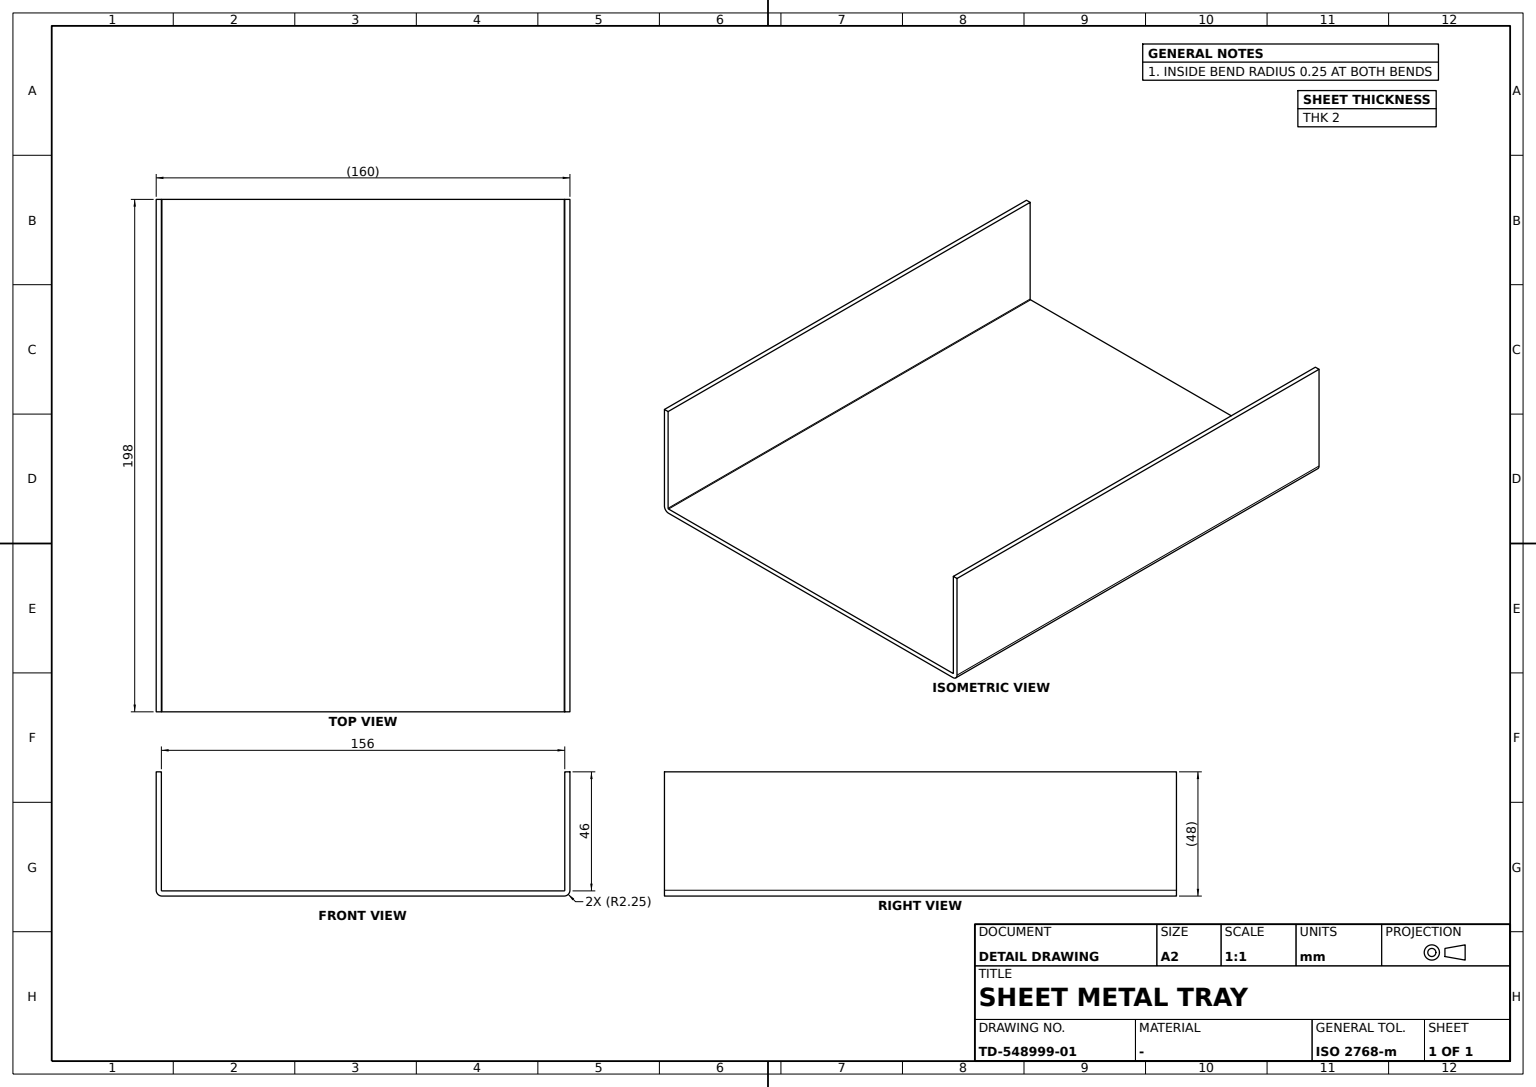
ISO-10303-21;
HEADER;
FILE_DESCRIPTION((''),'2;1');
FILE_NAME('','',(''),(''),'','','');
FILE_SCHEMA(('AUTOMOTIVE_DESIGN'));
ENDSEC;
DATA;
#1=APPLICATION_CONTEXT('');
#2=PRODUCT_CONTEXT('',#1,'mechanical');
#3=PRODUCT('','','',(#2));
#4=PRODUCT_DEFINITION_FORMATION('','',#3);
#5=PRODUCT_DEFINITION_CONTEXT('',#1,'design');
#6=PRODUCT_DEFINITION('','',#4,#5);
#7=PRODUCT_DEFINITION_SHAPE('','',#6);
#8=(LENGTH_UNIT()NAMED_UNIT(*)SI_UNIT(.MILLI.,.METRE.));
#9=(NAMED_UNIT(*)PLANE_ANGLE_UNIT()SI_UNIT($,.RADIAN.));
#10=(NAMED_UNIT(*)SI_UNIT($,.STERADIAN.)SOLID_ANGLE_UNIT());
#11=UNCERTAINTY_MEASURE_WITH_UNIT(LENGTH_MEASURE(1.E-05),#8,'distance_accuracy_value','');
#12=(GEOMETRIC_REPRESENTATION_CONTEXT(3)GLOBAL_UNCERTAINTY_ASSIGNED_CONTEXT((#11))GLOBAL_UNIT_ASSIGNED_CONTEXT((#8,#9,#10))REPRESENTATION_CONTEXT('',''));
#13=CARTESIAN_POINT('',(-77.75,-99.,0.));
#14=VERTEX_POINT('',#13);
#15=CARTESIAN_POINT('',(-80.,-99.,2.25));
#16=VERTEX_POINT('',#15);
#17=CARTESIAN_POINT('',(-77.75,-99.,2.25));
#18=DIRECTION('',(0.,1.,0.));
#19=DIRECTION('',(0.,0.,-1.));
#20=AXIS2_PLACEMENT_3D('',#17,#18,#19);
#21=CIRCLE('',#20,2.25);
#22=EDGE_CURVE('',#14,#16,#21,.T.);
#23=ORIENTED_EDGE('',*,*,#22,.F.);
#24=CARTESIAN_POINT('',(-77.75,-99.,2.));
#25=VERTEX_POINT('',#24);
#26=CARTESIAN_POINT('',(-77.75,-99.,1.));
#27=DIRECTION('',(0.,0.,1.));
#28=VECTOR('',#27,1000.);
#29=LINE('',#26,#28);
#30=EDGE_CURVE('',#14,#25,#29,.T.);
#31=ORIENTED_EDGE('',*,*,#30,.T.);
#32=CARTESIAN_POINT('',(-78.,-99.,2.25));
#33=VERTEX_POINT('',#32);
#34=CIRCLE('',#20,0.25);
#35=EDGE_CURVE('',#25,#33,#34,.T.);
#36=ORIENTED_EDGE('',*,*,#35,.T.);
#37=CARTESIAN_POINT('',(-79.,-99.,2.25));
#38=DIRECTION('',(1.,0.,0.));
#39=VECTOR('',#38,1000.);
#40=LINE('',#37,#39);
#41=EDGE_CURVE('',#16,#33,#40,.T.);
#42=ORIENTED_EDGE('',*,*,#41,.F.);
#43=EDGE_LOOP('',(#23,#31,#36,#42));
#44=FACE_OUTER_BOUND('',#43,.T.);
#45=CARTESIAN_POINT('',(-77.797124,-99.,2.));
#46=CARTESIAN_POINT('',(-78.174115,-99.,0.));
#47=CARTESIAN_POINT('',(-77.84425,-99.,2.011098));
#48=CARTESIAN_POINT('',(-78.59825,-99.,0.099885));
#49=CARTESIAN_POINT('',(-77.887876,-99.,2.03333));
#50=CARTESIAN_POINT('',(-78.990881,-99.,0.299966));
#51=CARTESIAN_POINT('',(-77.949009,-99.,2.085996));
#52=CARTESIAN_POINT('',(-79.541079,-99.,0.773968));
#53=CARTESIAN_POINT('',(-77.985194,-99.,2.156785));
#54=CARTESIAN_POINT('',(-79.866749,-99.,1.411067));
#55=CARTESIAN_POINT('',(-77.995066,-99.,2.187168));
#56=CARTESIAN_POINT('',(-79.955592,-99.,1.684512));
#57=CARTESIAN_POINT('',(-78.,-99.,2.218584));
#58=CARTESIAN_POINT('',(-80.,-99.,1.967257));
#59=B_SPLINE_SURFACE_WITH_KNOTS('',5,1,((#24,#13),(#45,#46),(#47,#48),(#49,#50),(#51,#52),(#53,#54),(#55,#56),(#57,#58),(#32,#15)),.UNSPECIFIED.,.F.,.F.,.F.,(6,3,6),(2,2),(0.,2.120575041,3.534291735),(-2.,0.),.UNSPECIFIED.);
#60=ADVANCED_FACE('',(#44),#59,.T.);
#61=CARTESIAN_POINT('',(80.,99.,2.25));
#62=VERTEX_POINT('',#61);
#63=CARTESIAN_POINT('',(78.,99.,2.25));
#64=VERTEX_POINT('',#63);
#65=CARTESIAN_POINT('',(79.,99.,2.25));
#66=DIRECTION('',(-1.,0.,0.));
#67=VECTOR('',#66,1000.);
#68=LINE('',#65,#67);
#69=EDGE_CURVE('',#62,#64,#68,.T.);
#70=ORIENTED_EDGE('',*,*,#69,.T.);
#71=CARTESIAN_POINT('',(78.,99.,48.));
#72=VERTEX_POINT('',#71);
#73=CARTESIAN_POINT('',(78.,99.,25.125));
#74=LINE('',#73,#28);
#75=EDGE_CURVE('',#64,#72,#74,.T.);
#76=ORIENTED_EDGE('',*,*,#75,.T.);
#77=CARTESIAN_POINT('',(80.,99.,48.));
#78=VERTEX_POINT('',#77);
#79=CARTESIAN_POINT('',(79.,99.,48.));
#80=LINE('',#79,#67);
#81=EDGE_CURVE('',#78,#72,#80,.T.);
#82=ORIENTED_EDGE('',*,*,#81,.F.);
#83=CARTESIAN_POINT('',(80.,99.,25.125));
#84=LINE('',#83,#28);
#85=EDGE_CURVE('',#62,#78,#84,.T.);
#86=ORIENTED_EDGE('',*,*,#85,.F.);
#87=EDGE_LOOP('',(#70,#76,#82,#86));
#88=FACE_OUTER_BOUND('',#87,.T.);
#89=CARTESIAN_POINT('',(78.,99.,2.));
#90=AXIS2_PLACEMENT_3D('',#89,#18,#27);
#91=PLANE('',#90);
#92=ADVANCED_FACE('',(#88),#91,.T.);
#93=CARTESIAN_POINT('',(-78.,99.,2.25));
#94=VERTEX_POINT('',#93);
#95=CARTESIAN_POINT('',(-78.,0.,2.25));
#96=DIRECTION('',(0.,-1.,0.));
#97=VECTOR('',#96,1000.);
#98=LINE('',#95,#97);
#99=EDGE_CURVE('',#94,#33,#98,.T.);
#100=ORIENTED_EDGE('',*,*,#99,.T.);
#101=ORIENTED_EDGE('',*,*,#35,.F.);
#102=CARTESIAN_POINT('',(-77.75,99.,2.));
#103=VERTEX_POINT('',#102);
#104=CARTESIAN_POINT('',(-77.75,0.,2.));
#105=VECTOR('',#18,1000.);
#106=LINE('',#104,#105);
#107=EDGE_CURVE('',#25,#103,#106,.T.);
#108=ORIENTED_EDGE('',*,*,#107,.T.);
#109=CARTESIAN_POINT('',(-77.75,99.,2.25));
#110=AXIS2_PLACEMENT_3D('',#109,#96,#19);
#111=CIRCLE('',#110,0.25);
#112=EDGE_CURVE('',#94,#103,#111,.T.);
#113=ORIENTED_EDGE('',*,*,#112,.F.);
#114=EDGE_LOOP('',(#100,#101,#108,#113));
#115=FACE_OUTER_BOUND('',#114,.T.);
#116=CARTESIAN_POINT('',(-77.75,0.,2.25));
#117=AXIS2_PLACEMENT_3D('',#116,#18,#19);
#118=CYLINDRICAL_SURFACE('',#117,0.25);
#119=ADVANCED_FACE('',(#115),#118,.F.);
#120=CARTESIAN_POINT('',(80.,-99.,2.25));
#121=VERTEX_POINT('',#120);
#122=CARTESIAN_POINT('',(77.75,-99.,0.));
#123=VERTEX_POINT('',#122);
#124=CARTESIAN_POINT('',(77.75,-99.,2.25));
#125=AXIS2_PLACEMENT_3D('',#124,#18,#38);
#126=CIRCLE('',#125,2.25);
#127=EDGE_CURVE('',#121,#123,#126,.T.);
#128=ORIENTED_EDGE('',*,*,#127,.F.);
#129=CARTESIAN_POINT('',(78.,-99.,2.25));
#130=VERTEX_POINT('',#129);
#131=CARTESIAN_POINT('',(79.,-99.,2.25));
#132=LINE('',#131,#67);
#133=EDGE_CURVE('',#121,#130,#132,.T.);
#134=ORIENTED_EDGE('',*,*,#133,.T.);
#135=CARTESIAN_POINT('',(77.75,-99.,2.));
#136=VERTEX_POINT('',#135);
#137=CIRCLE('',#125,0.25);
#138=EDGE_CURVE('',#130,#136,#137,.T.);
#139=ORIENTED_EDGE('',*,*,#138,.T.);
#140=CARTESIAN_POINT('',(77.75,-99.,1.));
#141=LINE('',#140,#28);
#142=EDGE_CURVE('',#123,#136,#141,.T.);
#143=ORIENTED_EDGE('',*,*,#142,.F.);
#144=EDGE_LOOP('',(#128,#134,#139,#143));
#145=FACE_OUTER_BOUND('',#144,.T.);
#146=CARTESIAN_POINT('',(78.,-99.,2.202876));
#147=CARTESIAN_POINT('',(80.,-99.,1.825885));
#148=CARTESIAN_POINT('',(77.988902,-99.,2.15575));
#149=CARTESIAN_POINT('',(79.900115,-99.,1.40175));
#150=CARTESIAN_POINT('',(77.96667,-99.,2.112124));
#151=CARTESIAN_POINT('',(79.700034,-99.,1.009119));
#152=CARTESIAN_POINT('',(77.914004,-99.,2.050991));
#153=CARTESIAN_POINT('',(79.226032,-99.,0.458921));
#154=CARTESIAN_POINT('',(77.843215,-99.,2.014806));
#155=CARTESIAN_POINT('',(78.588933,-99.,0.133251));
#156=CARTESIAN_POINT('',(77.812832,-99.,2.004934));
#157=CARTESIAN_POINT('',(78.315488,-99.,0.044408));
#158=CARTESIAN_POINT('',(77.781416,-99.,2.));
#159=CARTESIAN_POINT('',(78.032743,-99.,0.));
#160=B_SPLINE_SURFACE_WITH_KNOTS('',5,1,((#129,#120),(#146,#147),(#148,#149),(#150,#151),(#152,#153),(#154,#155),(#156,#157),(#158,#159),(#135,#122)),.UNSPECIFIED.,.F.,.F.,.F.,(6,3,6),(2,2),(0.,2.120575041,3.534291735),(-2.,0.),.UNSPECIFIED.);
#161=ADVANCED_FACE('',(#145),#160,.T.);
#162=CARTESIAN_POINT('',(80.,-99.,48.));
#163=VERTEX_POINT('',#162);
#164=CARTESIAN_POINT('',(80.,-99.,25.125));
#165=VECTOR('',#19,1000.);
#166=LINE('',#164,#165);
#167=EDGE_CURVE('',#163,#121,#166,.T.);
#168=ORIENTED_EDGE('',*,*,#167,.T.);
#169=CARTESIAN_POINT('',(80.,0.,2.25));
#170=LINE('',#169,#105);
#171=EDGE_CURVE('',#121,#62,#170,.T.);
#172=ORIENTED_EDGE('',*,*,#171,.T.);
#173=ORIENTED_EDGE('',*,*,#85,.T.);
#174=CARTESIAN_POINT('',(80.,0.,48.));
#175=LINE('',#174,#105);
#176=EDGE_CURVE('',#163,#78,#175,.T.);
#177=ORIENTED_EDGE('',*,*,#176,.F.);
#178=EDGE_LOOP('',(#168,#172,#173,#177));
#179=FACE_OUTER_BOUND('',#178,.T.);
#180=CARTESIAN_POINT('',(80.,0.,0.));
#181=AXIS2_PLACEMENT_3D('',#180,#38,#18);
#182=PLANE('',#181);
#183=ADVANCED_FACE('',(#179),#182,.T.);
#184=CARTESIAN_POINT('',(-78.,-99.,48.));
#185=VERTEX_POINT('',#184);
#186=CARTESIAN_POINT('',(-80.,-99.,48.));
#187=VERTEX_POINT('',#186);
#188=CARTESIAN_POINT('',(-79.,-99.,48.));
#189=LINE('',#188,#67);
#190=EDGE_CURVE('',#185,#187,#189,.T.);
#191=ORIENTED_EDGE('',*,*,#190,.T.);
#192=CARTESIAN_POINT('',(-80.,-99.,25.125));
#193=LINE('',#192,#28);
#194=EDGE_CURVE('',#16,#187,#193,.T.);
#195=ORIENTED_EDGE('',*,*,#194,.F.);
#196=ORIENTED_EDGE('',*,*,#41,.T.);
#197=CARTESIAN_POINT('',(-78.,-99.,25.125));
#198=LINE('',#197,#28);
#199=EDGE_CURVE('',#33,#185,#198,.T.);
#200=ORIENTED_EDGE('',*,*,#199,.T.);
#201=EDGE_LOOP('',(#191,#195,#196,#200));
#202=FACE_OUTER_BOUND('',#201,.T.);
#203=CARTESIAN_POINT('',(78.,-99.,48.));
#204=AXIS2_PLACEMENT_3D('',#203,#96,#19);
#205=PLANE('',#204);
#206=ADVANCED_FACE('',(#202),#205,.T.);
#207=ORIENTED_EDGE('',*,*,#133,.F.);
#208=ORIENTED_EDGE('',*,*,#167,.F.);
#209=VERTEX_POINT('',#203);
#210=CARTESIAN_POINT('',(79.,-99.,48.));
#211=LINE('',#210,#39);
#212=EDGE_CURVE('',#209,#163,#211,.T.);
#213=ORIENTED_EDGE('',*,*,#212,.F.);
#214=CARTESIAN_POINT('',(78.,-99.,25.125));
#215=LINE('',#214,#165);
#216=EDGE_CURVE('',#209,#130,#215,.T.);
#217=ORIENTED_EDGE('',*,*,#216,.T.);
#218=EDGE_LOOP('',(#207,#208,#213,#217));
#219=FACE_OUTER_BOUND('',#218,.T.);
#220=ADVANCED_FACE('',(#219),#205,.T.);
#221=CARTESIAN_POINT('',(78.,0.,2.25));
#222=LINE('',#221,#105);
#223=EDGE_CURVE('',#130,#64,#222,.T.);
#224=ORIENTED_EDGE('',*,*,#223,.F.);
#225=ORIENTED_EDGE('',*,*,#216,.F.);
#226=CARTESIAN_POINT('',(78.,0.,48.));
#227=LINE('',#226,#97);
#228=EDGE_CURVE('',#72,#209,#227,.T.);
#229=ORIENTED_EDGE('',*,*,#228,.F.);
#230=ORIENTED_EDGE('',*,*,#75,.F.);
#231=EDGE_LOOP('',(#224,#225,#229,#230));
#232=FACE_OUTER_BOUND('',#231,.T.);
#233=CARTESIAN_POINT('',(78.,0.,0.));
#234=AXIS2_PLACEMENT_3D('',#233,#38,#18);
#235=PLANE('',#234);
#236=ADVANCED_FACE('',(#232),#235,.F.);
#237=ORIENTED_EDGE('',*,*,#171,.F.);
#238=ORIENTED_EDGE('',*,*,#127,.T.);
#239=CARTESIAN_POINT('',(77.75,99.,0.));
#240=VERTEX_POINT('',#239);
#241=CARTESIAN_POINT('',(77.75,0.,0.));
#242=LINE('',#241,#97);
#243=EDGE_CURVE('',#240,#123,#242,.T.);
#244=ORIENTED_EDGE('',*,*,#243,.F.);
#245=CARTESIAN_POINT('',(77.75,99.,2.25));
#246=AXIS2_PLACEMENT_3D('',#245,#96,#38);
#247=CIRCLE('',#246,2.25);
#248=EDGE_CURVE('',#240,#62,#247,.T.);
#249=ORIENTED_EDGE('',*,*,#248,.T.);
#250=EDGE_LOOP('',(#237,#238,#244,#249));
#251=FACE_OUTER_BOUND('',#250,.T.);
#252=CARTESIAN_POINT('',(77.75,0.,2.25));
#253=AXIS2_PLACEMENT_3D('',#252,#18,#38);
#254=CYLINDRICAL_SURFACE('',#253,2.25);
#255=ADVANCED_FACE('',(#251),#254,.T.);
#256=CARTESIAN_POINT('',(-78.,99.,48.));
#257=VERTEX_POINT('',#256);
#258=CARTESIAN_POINT('',(-78.,99.,25.125));
#259=LINE('',#258,#165);
#260=EDGE_CURVE('',#257,#94,#259,.T.);
#261=ORIENTED_EDGE('',*,*,#260,.T.);
#262=CARTESIAN_POINT('',(-80.,99.,2.25));
#263=VERTEX_POINT('',#262);
#264=CARTESIAN_POINT('',(-79.,99.,2.25));
#265=LINE('',#264,#39);
#266=EDGE_CURVE('',#263,#94,#265,.T.);
#267=ORIENTED_EDGE('',*,*,#266,.F.);
#268=CARTESIAN_POINT('',(-80.,99.,48.));
#269=VERTEX_POINT('',#268);
#270=CARTESIAN_POINT('',(-80.,99.,25.125));
#271=LINE('',#270,#165);
#272=EDGE_CURVE('',#269,#263,#271,.T.);
#273=ORIENTED_EDGE('',*,*,#272,.F.);
#274=CARTESIAN_POINT('',(-79.,99.,48.));
#275=LINE('',#274,#39);
#276=EDGE_CURVE('',#269,#257,#275,.T.);
#277=ORIENTED_EDGE('',*,*,#276,.T.);
#278=EDGE_LOOP('',(#261,#267,#273,#277));
#279=FACE_OUTER_BOUND('',#278,.T.);
#280=ADVANCED_FACE('',(#279),#91,.T.);
#281=CARTESIAN_POINT('',(-77.75,99.,0.));
#282=VERTEX_POINT('',#281);
#283=CIRCLE('',#110,2.25);
#284=EDGE_CURVE('',#263,#282,#283,.T.);
#285=ORIENTED_EDGE('',*,*,#284,.T.);
#286=CARTESIAN_POINT('',(-77.75,0.,0.));
#287=LINE('',#286,#105);
#288=EDGE_CURVE('',#14,#282,#287,.T.);
#289=ORIENTED_EDGE('',*,*,#288,.F.);
#290=ORIENTED_EDGE('',*,*,#22,.T.);
#291=CARTESIAN_POINT('',(-80.,0.,2.25));
#292=LINE('',#291,#97);
#293=EDGE_CURVE('',#263,#16,#292,.T.);
#294=ORIENTED_EDGE('',*,*,#293,.F.);
#295=EDGE_LOOP('',(#285,#289,#290,#294));
#296=FACE_OUTER_BOUND('',#295,.T.);
#297=CYLINDRICAL_SURFACE('',#117,2.25);
#298=ADVANCED_FACE('',(#296),#297,.T.);
#299=ORIENTED_EDGE('',*,*,#243,.T.);
#300=CARTESIAN_POINT('',(0.,-99.,0.));
#301=LINE('',#300,#39);
#302=EDGE_CURVE('',#14,#123,#301,.T.);
#303=ORIENTED_EDGE('',*,*,#302,.F.);
#304=ORIENTED_EDGE('',*,*,#288,.T.);
#305=CARTESIAN_POINT('',(0.,99.,0.));
#306=LINE('',#305,#67);
#307=EDGE_CURVE('',#240,#282,#306,.T.);
#308=ORIENTED_EDGE('',*,*,#307,.F.);
#309=EDGE_LOOP('',(#299,#303,#304,#308));
#310=FACE_OUTER_BOUND('',#309,.T.);
#311=CARTESIAN_POINT('',(0.,0.,0.));
#312=AXIS2_PLACEMENT_3D('',#311,#27,#18);
#313=PLANE('',#312);
#314=ADVANCED_FACE('',(#310),#313,.F.);
#315=ORIENTED_EDGE('',*,*,#223,.T.);
#316=CARTESIAN_POINT('',(77.75,99.,2.));
#317=VERTEX_POINT('',#316);
#318=CIRCLE('',#246,0.25);
#319=EDGE_CURVE('',#317,#64,#318,.T.);
#320=ORIENTED_EDGE('',*,*,#319,.F.);
#321=CARTESIAN_POINT('',(77.75,0.,2.));
#322=LINE('',#321,#97);
#323=EDGE_CURVE('',#317,#136,#322,.T.);
#324=ORIENTED_EDGE('',*,*,#323,.T.);
#325=ORIENTED_EDGE('',*,*,#138,.F.);
#326=EDGE_LOOP('',(#315,#320,#324,#325));
#327=FACE_OUTER_BOUND('',#326,.T.);
#328=CYLINDRICAL_SURFACE('',#253,0.25);
#329=ADVANCED_FACE('',(#327),#328,.F.);
#330=ORIENTED_EDGE('',*,*,#190,.F.);
#331=CARTESIAN_POINT('',(-78.,0.,48.));
#332=LINE('',#331,#97);
#333=EDGE_CURVE('',#257,#185,#332,.T.);
#334=ORIENTED_EDGE('',*,*,#333,.F.);
#335=ORIENTED_EDGE('',*,*,#276,.F.);
#336=CARTESIAN_POINT('',(-80.,0.,48.));
#337=LINE('',#336,#105);
#338=EDGE_CURVE('',#187,#269,#337,.T.);
#339=ORIENTED_EDGE('',*,*,#338,.F.);
#340=EDGE_LOOP('',(#330,#334,#335,#339));
#341=FACE_OUTER_BOUND('',#340,.T.);
#342=AXIS2_PLACEMENT_3D('',#71,#27,#96);
#343=PLANE('',#342);
#344=ADVANCED_FACE('',(#341),#343,.T.);
#345=CARTESIAN_POINT('',(0.,-99.,2.));
#346=LINE('',#345,#39);
#347=EDGE_CURVE('',#25,#136,#346,.T.);
#348=ORIENTED_EDGE('',*,*,#347,.F.);
#349=ORIENTED_EDGE('',*,*,#30,.F.);
#350=ORIENTED_EDGE('',*,*,#302,.T.);
#351=ORIENTED_EDGE('',*,*,#142,.T.);
#352=EDGE_LOOP('',(#348,#349,#350,#351));
#353=FACE_OUTER_BOUND('',#352,.T.);
#354=CARTESIAN_POINT('',(-78.,-99.,0.));
#355=AXIS2_PLACEMENT_3D('',#354,#96,#38);
#356=PLANE('',#355);
#357=ADVANCED_FACE('',(#353),#356,.T.);
#358=ORIENTED_EDGE('',*,*,#338,.T.);
#359=ORIENTED_EDGE('',*,*,#272,.T.);
#360=ORIENTED_EDGE('',*,*,#293,.T.);
#361=ORIENTED_EDGE('',*,*,#194,.T.);
#362=EDGE_LOOP('',(#358,#359,#360,#361));
#363=FACE_OUTER_BOUND('',#362,.T.);
#364=CARTESIAN_POINT('',(-80.,0.,0.));
#365=AXIS2_PLACEMENT_3D('',#364,#38,#18);
#366=PLANE('',#365);
#367=ADVANCED_FACE('',(#363),#366,.F.);
#368=ORIENTED_EDGE('',*,*,#347,.T.);
#369=ORIENTED_EDGE('',*,*,#323,.F.);
#370=CARTESIAN_POINT('',(0.,99.,2.));
#371=LINE('',#370,#67);
#372=EDGE_CURVE('',#317,#103,#371,.T.);
#373=ORIENTED_EDGE('',*,*,#372,.T.);
#374=ORIENTED_EDGE('',*,*,#107,.F.);
#375=EDGE_LOOP('',(#368,#369,#373,#374));
#376=FACE_OUTER_BOUND('',#375,.T.);
#377=CARTESIAN_POINT('',(0.,0.,2.));
#378=AXIS2_PLACEMENT_3D('',#377,#27,#18);
#379=PLANE('',#378);
#380=ADVANCED_FACE('',(#376),#379,.T.);
#381=ORIENTED_EDGE('',*,*,#372,.F.);
#382=CARTESIAN_POINT('',(77.75,99.,1.));
#383=LINE('',#382,#28);
#384=EDGE_CURVE('',#240,#317,#383,.T.);
#385=ORIENTED_EDGE('',*,*,#384,.F.);
#386=ORIENTED_EDGE('',*,*,#307,.T.);
#387=CARTESIAN_POINT('',(-77.75,99.,1.));
#388=LINE('',#387,#28);
#389=EDGE_CURVE('',#282,#103,#388,.T.);
#390=ORIENTED_EDGE('',*,*,#389,.T.);
#391=EDGE_LOOP('',(#381,#385,#386,#390));
#392=FACE_OUTER_BOUND('',#391,.T.);
#393=CARTESIAN_POINT('',(78.,99.,0.));
#394=AXIS2_PLACEMENT_3D('',#393,#18,#66);
#395=PLANE('',#394);
#396=ADVANCED_FACE('',(#392),#395,.T.);
#397=ORIENTED_EDGE('',*,*,#81,.T.);
#398=ORIENTED_EDGE('',*,*,#228,.T.);
#399=ORIENTED_EDGE('',*,*,#212,.T.);
#400=ORIENTED_EDGE('',*,*,#176,.T.);
#401=EDGE_LOOP('',(#397,#398,#399,#400));
#402=FACE_OUTER_BOUND('',#401,.T.);
#403=ADVANCED_FACE('',(#402),#343,.T.);
#404=ORIENTED_EDGE('',*,*,#199,.F.);
#405=ORIENTED_EDGE('',*,*,#99,.F.);
#406=ORIENTED_EDGE('',*,*,#260,.F.);
#407=ORIENTED_EDGE('',*,*,#333,.T.);
#408=EDGE_LOOP('',(#404,#405,#406,#407));
#409=FACE_OUTER_BOUND('',#408,.T.);
#410=CARTESIAN_POINT('',(-78.,0.,0.));
#411=AXIS2_PLACEMENT_3D('',#410,#38,#18);
#412=PLANE('',#411);
#413=ADVANCED_FACE('',(#409),#412,.T.);
#414=ORIENTED_EDGE('',*,*,#248,.F.);
#415=ORIENTED_EDGE('',*,*,#384,.T.);
#416=ORIENTED_EDGE('',*,*,#319,.T.);
#417=ORIENTED_EDGE('',*,*,#69,.F.);
#418=EDGE_LOOP('',(#414,#415,#416,#417));
#419=FACE_OUTER_BOUND('',#418,.T.);
#420=CARTESIAN_POINT('',(78.,99.,2.202876));
#421=CARTESIAN_POINT('',(80.,99.,1.825885));
#422=CARTESIAN_POINT('',(77.988902,99.,2.15575));
#423=CARTESIAN_POINT('',(79.900115,99.,1.40175));
#424=CARTESIAN_POINT('',(77.96667,99.,2.112124));
#425=CARTESIAN_POINT('',(79.700034,99.,1.009119));
#426=CARTESIAN_POINT('',(77.914004,99.,2.050991));
#427=CARTESIAN_POINT('',(79.226032,99.,0.458921));
#428=CARTESIAN_POINT('',(77.843215,99.,2.014806));
#429=CARTESIAN_POINT('',(78.588933,99.,0.133251));
#430=CARTESIAN_POINT('',(77.812832,99.,2.004934));
#431=CARTESIAN_POINT('',(78.315488,99.,0.044408));
#432=CARTESIAN_POINT('',(77.781416,99.,2.));
#433=CARTESIAN_POINT('',(78.032743,99.,0.));
#434=B_SPLINE_SURFACE_WITH_KNOTS('',5,1,((#63,#61),(#420,#421),(#422,#423),(#424,#425),(#426,#427),(#428,#429),(#430,#431),(#432,#433),(#316,#239)),.UNSPECIFIED.,.F.,.F.,.F.,(6,3,6),(2,2),(0.,2.120575041,3.534291735),(-2.,0.),.UNSPECIFIED.);
#435=ADVANCED_FACE('',(#419),#434,.F.);
#436=ORIENTED_EDGE('',*,*,#112,.T.);
#437=ORIENTED_EDGE('',*,*,#389,.F.);
#438=ORIENTED_EDGE('',*,*,#284,.F.);
#439=ORIENTED_EDGE('',*,*,#266,.T.);
#440=EDGE_LOOP('',(#436,#437,#438,#439));
#441=FACE_OUTER_BOUND('',#440,.T.);
#442=CARTESIAN_POINT('',(-77.797124,99.,2.));
#443=CARTESIAN_POINT('',(-78.174115,99.,0.));
#444=CARTESIAN_POINT('',(-77.84425,99.,2.011098));
#445=CARTESIAN_POINT('',(-78.59825,99.,0.099885));
#446=CARTESIAN_POINT('',(-77.887876,99.,2.03333));
#447=CARTESIAN_POINT('',(-78.990881,99.,0.299966));
#448=CARTESIAN_POINT('',(-77.949009,99.,2.085996));
#449=CARTESIAN_POINT('',(-79.541079,99.,0.773968));
#450=CARTESIAN_POINT('',(-77.985194,99.,2.156785));
#451=CARTESIAN_POINT('',(-79.866749,99.,1.411067));
#452=CARTESIAN_POINT('',(-77.995066,99.,2.187168));
#453=CARTESIAN_POINT('',(-79.955592,99.,1.684512));
#454=CARTESIAN_POINT('',(-78.,99.,2.218584));
#455=CARTESIAN_POINT('',(-80.,99.,1.967257));
#456=B_SPLINE_SURFACE_WITH_KNOTS('',5,1,((#102,#281),(#442,#443),(#444,#445),(#446,#447),(#448,#449),(#450,#451),(#452,#453),(#454,#455),(#93,#262)),.UNSPECIFIED.,.F.,.F.,.F.,(6,3,6),(2,2),(0.,2.120575041,3.534291735),(-2.,0.),.UNSPECIFIED.);
#457=ADVANCED_FACE('',(#441),#456,.F.);
#458=CLOSED_SHELL('',(#60,#92,#119,#161,#183,#206,#220,#236,#255,#280,#298,#314,#329,#344,#357,#367,#380,#396,#403,#413,#435,#457));
#459=MANIFOLD_SOLID_BREP('',#458);
#460=ADVANCED_BREP_SHAPE_REPRESENTATION('',(#459),#12);
#461=SHAPE_DEFINITION_REPRESENTATION(#7,#460);
ENDSEC;
END-ISO-10303-21;
